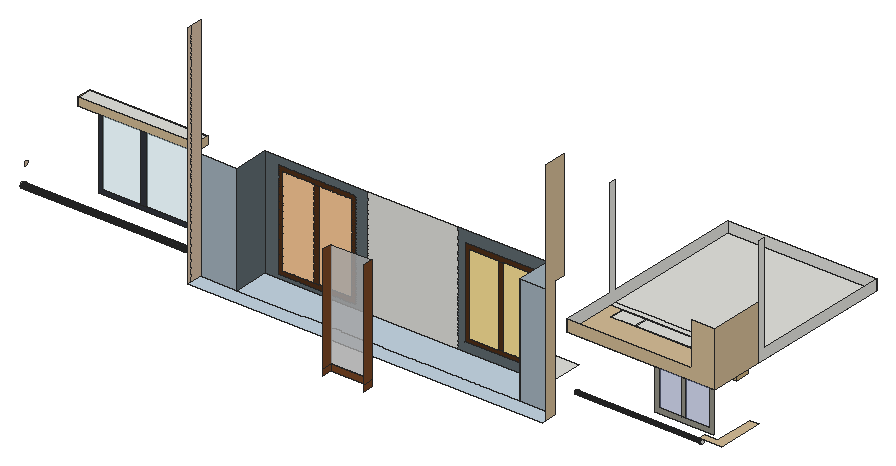
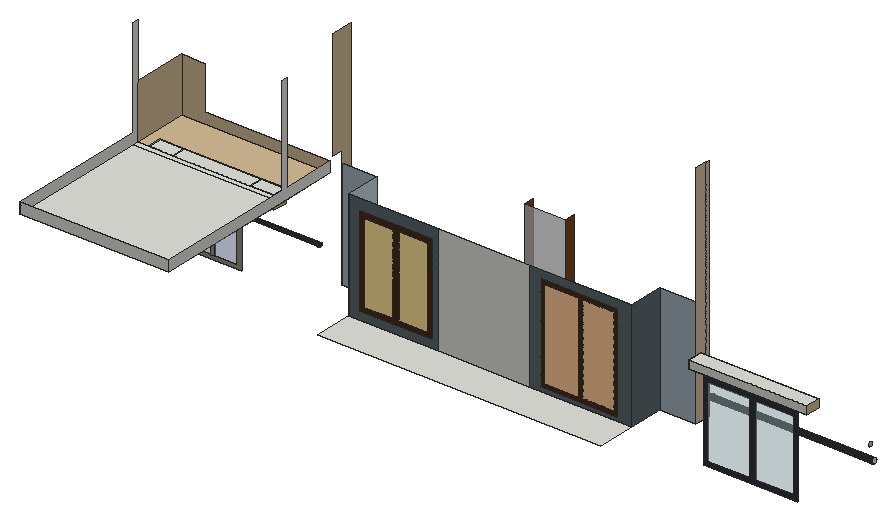
# SketchUp Ruby script. Lengths in inches.
U = 1.inch
M = Sketchup.active_model
def pt(a) = Geom::Point3d.new(a.map { |v| v * U })
def face(e, loops, mat)
  f = e.add_face(loops[0].map { |a| pt(a) })
  loops[1..].each { |l| e.add_face(l.map { |a| pt(a) }).erase! }
  f.material = f.back_material = mat if mat
  f
end
# faces: each face lists its corners as indices into pts; further lists are holes
def faces(e, pts, list, mat = nil) = list.each { |f| face(e, (f[0].is_a?(Array) ? f : [f]).map { |l| l.map { |i| pts[i] } }, mat) }
# xy, xz, yz: faces in a plane at the given z, y or x. An outline is a flat list of corners, or four numbers for a rectangle; further outlines are holes
def ring(l) = l.size == 4 ? [[l[0], l[1]], [l[2], l[1]], [l[2], l[3]], [l[0], l[3]]] : l.each_slice(2).to_a
def flat(e, list, mat, &to3) = list.each { |f| face(e, (f[0].is_a?(Array) ? f : [f]).map { |l| ring(l).map { |u, v| to3.(u, v) } }, mat) }
def xy(e, z, list, mat = nil) = flat(e, list, mat) { |x, y| [x, y, z] }
def xz(e, y, list, mat = nil) = flat(e, list, mat) { |x, z| [x, y, z] }
def yz(e, x, list, mat = nil) = flat(e, list, mat) { |y, z| [x, y, z] }
def lines(e, pts, list) = list.each { |a, b| e.add_line(pt(pts[a]), pt(pts[b])) }
# prism: a flat outline (further loops are holes) pulled along v
def prism(e, loops, v, mat = nil)
  f = face(e, loops, mat); d = Geom::Vector3d.new(v.map { |x| x * U })
  f.pushpull(f.normal.samedirection?(d) ? d.length : -d.length)
end
def box(e, o, s, mat = nil) = prism(e, [[o, [o[0] + s[0], o[1], o[2]], [o[0] + s[0], o[1] + s[1], o[2]], [o[0], o[1] + s[1], o[2]]]], [0, 0, s[2]], mat)
def at(x, y, z, deg = 0) = Geom::Transformation.translation(pt([x, y, z])) * Geom::Transformation.rotation(ORIGIN, Z_AXIS, deg.degrees)
def axes(o, x, y, z) = Geom::Transformation.new([*x, 0, *y, 0, *z, 0, *pt(o).to_a, 1])
def part(name) = M.definitions.add(name)
# library, detail: a bought-in or finely detailed component or shape, given as its bounding box
def library(name, o, s) = part(name).tap { |d| box(d.entities, o, s) }
def detail(e, o, s) = box(e.add_group.entities, o, s)
def put(e, d, t, mat = nil) = e.add_instance(d, t).tap { |i| i.material = mat if mat }
def group(e, t, mat = nil) = e.add_group.tap { |g| g.transformation = t; g.material = mat if mat }.entities
root = M.entities
M.materials.add("[Color C02]").color = [255, 204, 153]
M.materials.add("[Color D02]").color = [255, 229, 153]
M.materials.add("[Formica Beige]").color = [211, 187, 149]
M.materials.add("[Formica Graystone]").color = [149, 146, 135]
M.materials.add("[Formica Laminate Dark]").color = [50, 53, 60]
M.materials.add("[Formica Laminate Light]").color = [213, 189, 164]
M.materials.add("[Formica Speckled Grey]").color = [94, 105, 111]
M.materials.add("[Terrazzo Light Blue]1").color = [165, 180, 191]
M.materials.add("[Terrazzo Light Blue]2").color = [196, 214, 227]
M.materials.add("[Translucent Glass Safety]").color = [204, 235, 244]
M.materials["[Translucent Glass Safety]"].alpha = 0.5
M.materials.add("[Translucent Glass Sky Reflection]").color = [126, 138, 183]
M.materials["[Translucent Glass Sky Reflection]"].alpha = 0.52
M.materials.add("[Translucent Resin Crush Gray]").color = [201, 201, 201]
M.materials["[Translucent Resin Crush Gray]"].alpha = 0.8
M.materials.add("[Wood Floor Light]").color = [204, 176, 127]
M.materials.add("[Wood Veneer 01]").color = [79, 46, 24]
M.materials.add("[Wood Veneer 01]2").color = [120, 70, 37]
xy(root,393,[[238.58,174.4375,549.2,216.67]])
xy(root,393,[[198.57,119.07,588.3,135.71],[238.58,135.71,549.2,174.4375]],"[Terrazzo Light Blue]2")
xy(root,418,[[80.57,126.78,80.98,126.79,81.37,126.91,81.71,127.125,81.99,127.42,82.18,127.78,82.28,128.18,82.26,128.59,82.14,128.98,81.93,129.33,81.63,129.6,81.27,129.8,80.87,129.89,80.46,129.875,80.07,129.76,79.73,129.54,79.45,129.24,79.26,128.88,79.17,128.48,79.18,128.08,79.3,127.6875,79.51,127.34,79.8125,127.0625,80.17,126.87]])
xy(root,418.3125,[[52.63,126.78,53.04,126.79,53.43,126.91,53.78,127.125,54.05,127.42,54.25,127.78,54.34,128.18,54.32,128.59,54.21,128.98,53.99,129.33,53.69,129.6,53.33,129.8,52.93,129.89,52.53,129.875,52.14,129.76,51.79,129.54,51.51,129.24,51.32,128.88,51.23,128.48,51.24,128.08,51.36,127.6875,51.58,127.34,51.875,127.0625,52.23,126.87]])
xy(root,418.375,[[112.07,126.78,112.48,126.79,112.87,126.91,113.21,127.125,113.49,127.42,113.68,127.78,113.78,128.18,113.76,128.59,113.64,128.98,113.43,129.33,113.13,129.6,112.77,129.8,112.37,129.89,111.96,129.875,111.57,129.76,111.23,129.54,110.95,129.24,110.76,128.88,110.67,128.48,110.68,128.08,110.8,127.6875,111.01,127.34,111.3125,127.0625,111.67,126.87]])
xy(root,418.5625,[[139.32,126.78,139.73,126.79,140.12,126.91,140.46,127.125,140.74,127.42,140.93,127.78,141.03,128.18,141.01,128.59,140.89,128.98,140.68,129.33,140.38,129.6,140.02,129.8,139.62,129.89,139.21,129.875,138.82,129.76,138.48,129.54,138.2,129.24,138.01,128.88,137.92,128.48,137.93,128.08,138.05,127.6875,138.26,127.34,138.5625,127.0625,138.92,126.87]])
xy(root,418.625,[[13.88,126.78,14.29,126.79,14.68,126.91,15.03,127.125,15.3,127.42,15.5,127.78,15.59,128.18,15.57,128.59,15.46,128.98,15.24,129.33,14.94,129.6,14.58,129.8,14.18,129.89,13.78,129.875,13.39,129.76,13.04,129.54,12.76,129.24,12.57,128.88,12.48,128.48,12.49,128.08,12.61,127.6875,12.83,127.34,13.125,127.0625,13.48,126.87]])
xy(root,418.875,[[166.69,126.78,167.1,126.79,167.49,126.91,167.84,127.125,168.12,127.42,168.31,127.78,168.4,128.18,168.39,128.59,168.27,128.98,168.05,129.33,167.75,129.6,167.39,129.8,167,129.89,166.59,129.875,166.2,129.76,165.85,129.54,165.57,129.24,165.38,128.88,165.29,128.48,165.3,128.08,165.42,127.6875,165.64,127.34,165.9375,127.0625,166.3,126.87]])
xy(root,419.3125,[[95.76,126.78,96.16,126.79,96.55,126.91,96.9,127.125,97.18,127.42,97.37,127.78,97.46,128.18,97.45,128.59,97.33,128.98,97.11,129.33,96.82,129.6,96.46,129.8,96.06,129.89,95.65,129.875,95.26,129.76,94.92,129.54,94.64,129.24,94.44,128.88,94.35,128.48,94.37,128.08,94.49,127.6875,94.7,127.34,95,127.0625,95.36,126.87]])
xy(root,419.5,[[153.76,126.78,154.16,126.79,154.55,126.91,154.9,127.125,155.18,127.42,155.37,127.78,155.46,128.18,155.45,128.59,155.33,128.98,155.11,129.33,154.82,129.6,154.46,129.8,154.06,129.89,153.65,129.875,153.26,129.76,152.92,129.54,152.64,129.24,152.44,128.88,152.35,128.48,152.37,128.08,152.49,127.6875,152.7,127.34,153,127.0625,153.36,126.87]])
xy(root,419.75,[[125.44,126.78,125.85,126.79,126.24,126.91,126.59,127.125,126.87,127.42,127.06,127.78,127.15,128.18,127.14,128.59,127.02,128.98,126.8,129.33,126.5,129.6,126.14,129.8,125.75,129.89,125.34,129.875,124.95,129.76,124.6,129.54,124.32,129.24,124.13,128.88,124.04,128.48,124.05,128.08,124.17,127.6875,124.39,127.34,124.6875,127.0625,125.05,126.87]])
xy(root,420.0625,[[66.19,126.78,66.6,126.79,66.99,126.91,67.34,127.125,67.62,127.42,67.81,127.78,67.9,128.18,67.89,128.59,67.77,128.98,67.55,129.33,67.25,129.6,66.89,129.8,66.5,129.89,66.09,129.875,65.7,129.76,65.35,129.54,65.07,129.24,64.88,128.88,64.79,128.48,64.8,128.08,64.92,127.6875,65.14,127.34,65.4375,127.0625,65.8,126.87]])
xy(root,420.65,[[179.57,126.78,179.98,126.79,180.37,126.91,180.71,127.125,180.99,127.42,181.18,127.78,181.28,128.18,181.26,128.59,181.14,128.98,180.93,129.33,180.63,129.6,180.27,129.8,179.87,129.89,179.46,129.875,179.07,129.76,178.73,129.54,178.45,129.24,178.26,128.88,178.17,128.48,178.18,128.08,178.3,127.6875,178.51,127.34,178.8125,127.0625,179.17,126.87]])
xy(root,421.29,[[25.07,126.78,25.48,126.79,25.87,126.91,26.21,127.125,26.49,127.42,26.68,127.78,26.78,128.18,26.76,128.59,26.64,128.98,26.43,129.33,26.13,129.6,25.77,129.8,25.37,129.89,24.96,129.875,24.57,129.76,24.23,129.54,23.95,129.24,23.76,128.88,23.67,128.48,23.68,128.08,23.8,127.6875,24.01,127.34,24.3125,127.0625,24.67,126.87]])
xy(root,421.85,[[39.26,126.78,39.66,126.79,40.05,126.91,40.4,127.125,40.68,127.42,40.87,127.78,40.96,128.18,40.95,128.59,40.83,128.98,40.61,129.33,40.32,129.6,39.96,129.8,39.56,129.89,39.15,129.875,38.76,129.76,38.42,129.54,38.14,129.24,37.94,128.88,37.85,128.48,37.87,128.08,37.99,127.6875,38.2,127.34,38.5,127.0625,38.86,126.87]])
xy(root,422.625,[[730.9,134.27,731.27,134.32,731.62,134.46,731.92,134.6875,732.15,134.99,732.29,135.33,732.34,135.7,732.29,136.08,732.15,136.42,731.92,136.72,731.62,136.95,731.27,137.09,730.9,137.14,730.53,137.09,730.18,136.95,729.89,136.72,729.66,136.42,729.51,136.08,729.46,135.7,729.51,135.33,729.66,134.99,729.89,134.6875,730.18,134.46,730.53,134.32]])
xy(root,423.0625,[[742.96,134.27,743.34,134.32,743.68,134.46,743.98,134.6875,744.21,134.99,744.35,135.33,744.4,135.7,744.35,136.08,744.21,136.42,743.98,136.72,743.68,136.95,743.34,137.09,742.96,137.14,742.59,137.09,742.25,136.95,741.95,136.72,741.72,136.42,741.58,136.08,741.53,135.7,741.58,135.33,741.72,134.99,741.95,134.6875,742.25,134.46,742.59,134.32]])
xy(root,423.375,[[618.46,134.27,618.84,134.32,619.18,134.46,619.48,134.6875,619.71,134.99,619.85,135.33,619.9,135.7,619.85,136.08,619.71,136.42,619.48,136.72,619.18,136.95,618.84,137.09,618.46,137.14,618.09,137.09,617.75,136.95,617.45,136.72,617.22,136.42,617.08,136.08,617.03,135.7,617.08,135.33,617.22,134.99,617.45,134.6875,617.75,134.46,618.09,134.32]])
xy(root,423.6875,[[631.71,134.27,632.09,134.32,632.43,134.46,632.73,134.6875,632.96,134.99,633.1,135.33,633.15,135.7,633.1,136.08,632.96,136.42,632.73,136.72,632.43,136.95,632.09,137.09,631.71,137.14,631.34,137.09,631,136.95,630.7,136.72,630.47,136.42,630.33,136.08,630.28,135.7,630.33,135.33,630.47,134.99,630.7,134.6875,631,134.46,631.34,134.32]])
xy(root,423.75,[[697.03,134.27,697.4,134.32,697.75,134.46,698.04,134.6875,698.27,134.99,698.42,135.33,698.46,135.7,698.42,136.08,698.27,136.42,698.04,136.72,697.75,136.95,697.4,137.09,697.03,137.14,696.66,137.09,696.31,136.95,696.01,136.72,695.78,136.42,695.64,136.08,695.59,135.7,695.64,135.33,695.78,134.99,696.01,134.6875,696.31,134.46,696.66,134.32]])
xy(root,424.25,[[682.4,134.27,682.77,134.32,683.12,134.46,683.42,134.6875,683.65,134.99,683.79,135.33,683.84,135.7,683.79,136.08,683.65,136.42,683.42,136.72,683.12,136.95,682.77,137.09,682.4,137.14,682.03,137.09,681.68,136.95,681.39,136.72,681.16,136.42,681.01,136.08,680.96,135.7,681.01,135.33,681.16,134.99,681.39,134.6875,681.68,134.46,682.03,134.32]])
xy(root,424.375,[[647.4,134.27,647.77,134.32,648.12,134.46,648.42,134.6875,648.65,134.99,648.79,135.33,648.84,135.7,648.79,136.08,648.65,136.42,648.42,136.72,648.12,136.95,647.77,137.09,647.4,137.14,647.03,137.09,646.68,136.95,646.39,136.72,646.16,136.42,646.01,136.08,645.96,135.7,646.01,135.33,646.16,134.99,646.39,134.6875,646.68,134.46,647.03,134.32]])
xy(root,424.43,[[715.03,134.27,715.4,134.32,715.75,134.46,716.04,134.6875,716.27,134.99,716.42,135.33,716.46,135.7,716.42,136.08,716.27,136.42,716.04,136.72,715.75,136.95,715.4,137.09,715.03,137.14,714.66,137.09,714.31,136.95,714.01,136.72,713.78,136.42,713.64,136.08,713.59,135.7,713.64,135.33,713.78,134.99,714.01,134.6875,714.31,134.46,714.66,134.32]])
xy(root,424.8125,[[664.53,134.27,664.9,134.32,665.25,134.46,665.54,134.6875,665.77,134.99,665.92,135.33,665.96,135.7,665.92,136.08,665.77,136.42,665.54,136.72,665.25,136.95,664.9,137.09,664.53,137.14,664.16,137.09,663.81,136.95,663.51,136.72,663.28,136.42,663.14,136.08,663.09,135.7,663.14,135.33,663.28,134.99,663.51,134.6875,663.81,134.46,664.16,134.32]])
xy(root,429,[[750.32,131.74,774.15,131.74,774.15,182.57,764.43,182.57,764.43,138.95,750.32,138.95]],"[Formica Beige]")
xy(root,474.11,[[624.7,167.26,651.04,182.57],[735.89,167.26,762.23,182.57]])
xy(root,474.11,[[651.04,167.26,735.89,182.57]],"[Wood Floor Light]")
xy(root,484.63,[[32.67,175.33,161.92,191.15]],"[Formica Beige]")
xy(root,489,[[624.7,167.26,651.04,182.57],[651.04,167.26,735.89,182.57],[735.89,167.26,762.23,182.57],[611.125,182.57,774.15,189.24],[611.125,189.24,774.15,344.36]])
xy(root,489,[[611.125,122.79,611.125,182.57,624.7,182.57,624.7,167.26,762.23,167.26,762.23,182.57,774.15,182.57,774.15,122.79]],"[Formica Beige]")
xy(root,493.63,[[32.67,175.33,161.92,191.15]])
xz(root,88.2,[[380.3,390.9,424.94,508.89]],"[Translucent Resin Crush Gray]")
xz(root,88.2,[[380.3,384.08,424.94,390.9]],"[Wood Veneer 01]2")
xz(root,122.79,[[611.125,489,774.15,489,774.15,549,748.22,549,748.22,501,611.125,501]],"[Formica Beige]")
xz(root,135.71,[[198.57,393,238.58,513],[549.2,393,588.3,513]],"[Terrazzo Light Blue]1")
xz(root,167.26,[[624.7,474.11,651.04,489],[651.04,474.11,735.89,489],[735.89,474.11,762.23,489]],"[Wood Floor Light]")
xz(root,174.4375,[[351.88,393,450.54,513]])
xz(root,174.4375,[[258.23,402.07,291.74,499.58],[297.7,402.07,333.48,499.58]],"[Color C02]")
xz(root,174.4375,[[463.97,407.63,493.92,495.13],[501.09,407.63,531.22,495.13]],"[Color D02]")
xz(root,174.4375,[[[238.58,393,351.88,513],[253.32,397.17,338.39,504.48]],[[450.54,393,549.2,513],[458.41,402.07,536.78,500.6875]]],"[Formica Speckled Grey]")
xz(root,174.4375,[[[253.32,397.17,338.39,504.48],[258.23,402.07,333.48,499.58]],[291.74,402.07,297.7,499.58],[[458.41,402.07,536.78,500.6875],[463.97,407.63,531.22,495.13]],[493.92,407.63,501.09,495.13]],"[Wood Veneer 01]")
xz(root,175.33,[[32.67,484.63,161.92,493.63]],"[Formica Beige]")
xz(root,182.57,[[624.7,474.11,651.04,489],[651.04,474.11,735.89,489],[735.89,474.11,762.23,489]])
xz(root,182.57,[[[660.63,401.51,725.25,472.38],[665.45,406.33,720.43,467.5625]],[690.15,406.33,694.17,467.5625]],"[Formica Graystone]")
xz(root,182.57,[[665.45,406.33,690.15,467.5625],[694.17,406.33,720.43,467.5625]],"[Translucent Glass Sky Reflection]")
xz(root,191.15,[[32.67,484.63,161.92,493.63]])
xz(root,191.15,[[[42.1875,395.58,146.3125,483.45],[46.93,400.32,141.57,478.71]],[88.56,400.32,95.82,478.71]],"[Formica Laminate Dark]")
xz(root,191.15,[[46.93,400.32,88.56,478.71],[95.82,400.32,141.57,478.71]],"[Translucent Glass Safety]")
xz(root,344.36,[[611.125,489,774.15,501]])
yz(root,9,[[128.15,417.26,127.45,417.35,126.8,417.625,126.25,418.05,125.82,418.61,125.55,419.26,125.46,419.95,125.55,420.65,125.82,421.29,126.25,421.85,126.8,422.28,127.45,422.55,128.15,422.64,128.84,422.55,129.49,422.28,130.05,421.85,130.48,421.29,130.74,420.65,130.84,419.95,130.74,419.26,130.48,418.61,130.05,418.05,129.49,417.625,128.84,417.35]])
yz(root,9,[[133.36,436.53,132.81,436.61,132.3,436.82,131.86,437.16,131.52,437.6,131.31,438.11,131.23,438.66,131.31,439.21,131.52,439.72,131.86,440.16,132.3,440.5,132.81,440.71,133.36,440.78,133.91,440.71,134.42,440.5,134.86,440.16,135.2,439.72,135.41,439.21,135.48,438.66,135.41,438.11,135.2,437.6,134.86,437.16,134.42,436.82,133.91,436.61]],"[Formica Laminate Light]")
yz(root,32.67,[[175.33,484.63,191.15,493.63]],"[Formica Beige]")
yz(root,161.92,[[175.33,484.63,191.15,493.63]],"[Formica Beige]")
yz(root,198.57,[[119.07,393,122.79,645],[122.79,393,135.71,645]],"[Formica Laminate Light]")
yz(root,238.58,[[135.71,393,174.4375,513]],"[Formica Speckled Grey]")
yz(root,380.3,[[77.26,384.08,88.2,390.9],[77.26,390.9,88.2,508.89]],"[Wood Veneer 01]2")
yz(root,424.94,[[77.26,384.08,88.2,390.9],[77.26,390.9,88.2,508.89]],"[Wood Veneer 01]2")
yz(root,549.2,[[135.71,393,174.4375,513]],"[Terrazzo Light Blue]2")
yz(root,588.3,[[122.79,393,122.79,645,147.05,645,147.05,525,135.71,525,135.71,393]],"[Formica Beige]")
yz(root,611.125,[[122.79,489,344.36,489,344.36,501,189.24,501,189.24,609,182.57,609,182.57,501,122.79,501]])
yz(root,624.7,[[167.26,474.11,182.57,489]],"[Wood Floor Light]")
yz(root,651.04,[[167.26,474.11,182.57,489]])
yz(root,735.89,[[167.26,474.11,182.57,489]])
yz(root,750.32,[[135.46,422.23,135.91,422.29,136.33,422.46,136.7,422.74,136.98,423.1,137.15,423.53,137.21,423.98,137.15,424.43,136.98,424.85,136.7,425.22,136.33,425.49,135.91,425.67,135.46,425.73,135.01,425.67,134.58,425.49,134.22,425.22,133.94,424.85,133.77,424.43,133.71,423.98,133.77,423.53,133.94,423.1,134.22,422.74,134.58,422.46,135.01,422.29]])
yz(root,762.23,[[167.26,474.11,182.57,489]],"[Wood Floor Light]")
yz(root,774.15,[[182.57,489,182.57,609,189.24,609,189.24,501,344.36,501,344.36,489]])
yz(root,774.15,[[122.79,489,182.57,549]],"[Formica Beige]")
p = [[9,127.45,417.35],[9,128.15,417.26],[189.57,128.15,417.26],[189.57,127.45,417.35],[9,128.84,417.35],[189.57,128.84,417.35],
  [9,126.8,417.625],[189.57,126.8,417.625],[9,129.49,417.625],[189.57,129.49,417.625],[9,126.25,418.05],[189.57,126.25,418.05],
  [9,130.05,418.05],[189.57,130.05,418.05],[9,125.82,418.61],[189.57,125.82,418.61],[9,130.48,418.61],[189.57,130.48,418.61],
  [9,125.55,419.26],[189.57,125.55,419.26],[9,130.74,419.26],[189.57,130.74,419.26],[9,125.46,419.95],[189.57,125.46,419.95],
  [9,130.84,419.95],[189.57,130.84,419.95],[9,125.55,420.65],[189.57,125.55,420.65],[9,130.74,420.65],[189.57,130.74,420.65],
  [9,125.82,421.29],[189.57,125.82,421.29],[9,130.48,421.29],[189.57,130.48,421.29],[9,126.25,421.85],[189.57,126.25,421.85],
  [9,130.05,421.85],[189.57,130.05,421.85],[9,126.8,422.28],[189.57,126.8,422.28],[9,129.49,422.28],[189.57,129.49,422.28],
  [750.32,135.46,422.23],[750.32,135.01,422.29],[611.125,135.01,422.29],[611.125,135.46,422.23],[750.32,135.91,422.29],[611.125,135.91,422.29],
  [9,127.45,422.55],[189.57,127.45,422.55],[9,128.84,422.55],[189.57,128.84,422.55],[750.32,134.58,422.46],[611.125,134.58,422.46],
  [750.32,136.33,422.46],[611.125,136.33,422.46],[9,128.15,422.64],[189.57,128.15,422.64],[750.32,134.22,422.74],[611.125,134.22,422.74],
  [750.32,136.7,422.74],[611.125,136.7,422.74],[750.32,133.94,423.1],[611.125,133.94,423.1],[750.32,136.98,423.1],[611.125,136.98,423.1],
  [750.32,133.77,423.53],[611.125,133.77,423.53],[750.32,137.15,423.53],[611.125,137.15,423.53],[750.32,133.71,423.98],[611.125,133.71,423.98],
  [750.32,137.21,423.98],[611.125,137.21,423.98],[750.32,133.77,424.43],[611.125,133.77,424.43],[750.32,137.15,424.43],[611.125,137.15,424.43],
  [750.32,133.94,424.85],[611.125,133.94,424.85],[750.32,136.98,424.85],[611.125,136.98,424.85],[750.32,134.22,425.22],[611.125,134.22,425.22],
  [750.32,136.7,425.22],[611.125,136.7,425.22],[750.32,134.58,425.49],[611.125,134.58,425.49],[750.32,136.33,425.49],[611.125,136.33,425.49],
  [750.32,135.01,425.67],[611.125,135.01,425.67],[750.32,135.91,425.67],[611.125,135.91,425.67],[750.32,135.46,425.73],[611.125,135.46,425.73]]
faces(root,p,[[0,1,2,3],[1,4,5,2],[6,0,3,7],[4,8,9,5],[10,6,7,11],[8,12,13,9],[14,10,11,15],[12,16,17,13],
  [18,14,15,19],[16,20,21,17],[22,18,19,23],[20,24,25,21],[26,22,23,27],[24,28,29,25],[30,26,27,31],[28,32,33,29],
  [34,30,31,35],[32,36,37,33],[38,34,35,39],[36,40,41,37],[42,43,44,45],[46,42,45,47],[48,38,39,49],[40,50,51,41],
  [43,52,53,44],[54,46,47,55],[56,48,49,57],[50,56,57,51],[52,58,59,53],[60,54,55,61],[58,62,63,59],[64,60,61,65],
  [62,66,67,63],[68,64,65,69],[66,70,71,67],[72,68,69,73],[70,74,75,71],[76,72,73,77],[74,78,79,75],[80,76,77,81],
  [78,82,83,79],[84,80,81,85],[82,86,87,83],[88,84,85,89],[86,90,91,87],[92,88,89,93],[90,94,95,91],[94,92,93,95]],"[Formica Laminate Dark]")
